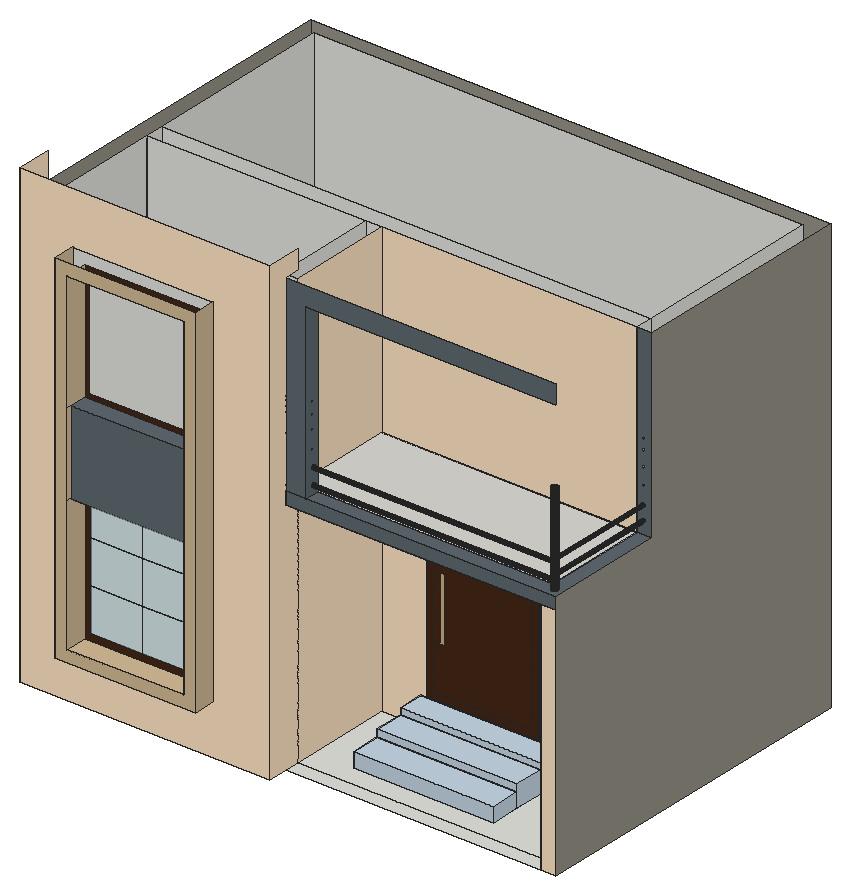
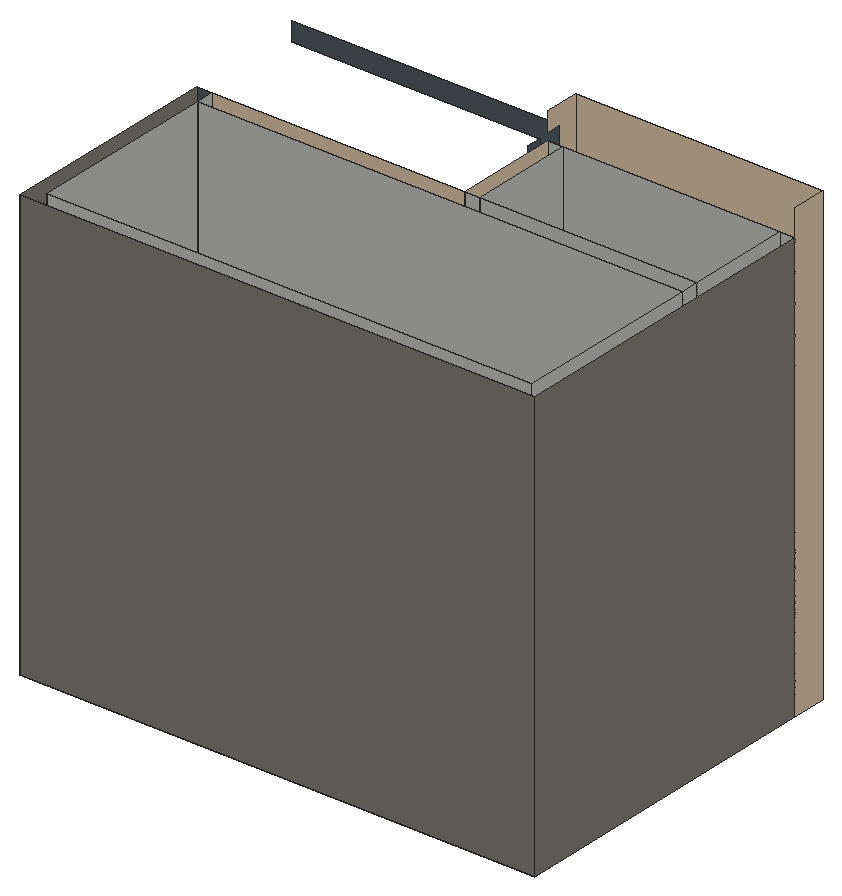
# SketchUp Ruby script. Lengths in inches.
U = 1.inch
M = Sketchup.active_model
def pt(a) = Geom::Point3d.new(a.map { |v| v * U })
def face(e, loops, mat)
  f = e.add_face(loops[0].map { |a| pt(a) })
  loops[1..].each { |l| e.add_face(l.map { |a| pt(a) }).erase! }
  f.material = f.back_material = mat if mat
  f
end
# faces: each face lists its corners as indices into pts; further lists are holes
def faces(e, pts, list, mat = nil) = list.each { |f| face(e, (f[0].is_a?(Array) ? f : [f]).map { |l| l.map { |i| pts[i] } }, mat) }
# xy, xz, yz: faces in a plane at the given z, y or x. An outline is a flat list of corners, or four numbers for a rectangle; further outlines are holes
def ring(l) = l.size == 4 ? [[l[0], l[1]], [l[2], l[1]], [l[2], l[3]], [l[0], l[3]]] : l.each_slice(2).to_a
def flat(e, list, mat, &to3) = list.each { |f| face(e, (f[0].is_a?(Array) ? f : [f]).map { |l| ring(l).map { |u, v| to3.(u, v) } }, mat) }
def xy(e, z, list, mat = nil) = flat(e, list, mat) { |x, y| [x, y, z] }
def xz(e, y, list, mat = nil) = flat(e, list, mat) { |x, z| [x, y, z] }
def yz(e, x, list, mat = nil) = flat(e, list, mat) { |y, z| [x, y, z] }
def lines(e, pts, list) = list.each { |a, b| e.add_line(pt(pts[a]), pt(pts[b])) }
# prism: a flat outline (further loops are holes) pulled along v
def prism(e, loops, v, mat = nil)
  f = face(e, loops, mat); d = Geom::Vector3d.new(v.map { |x| x * U })
  f.pushpull(f.normal.samedirection?(d) ? d.length : -d.length)
end
def box(e, o, s, mat = nil) = prism(e, [[o, [o[0] + s[0], o[1], o[2]], [o[0] + s[0], o[1] + s[1], o[2]], [o[0], o[1] + s[1], o[2]]]], [0, 0, s[2]], mat)
def at(x, y, z, deg = 0) = Geom::Transformation.translation(pt([x, y, z])) * Geom::Transformation.rotation(ORIGIN, Z_AXIS, deg.degrees)
def axes(o, x, y, z) = Geom::Transformation.new([*x, 0, *y, 0, *z, 0, *pt(o).to_a, 1])
def part(name) = M.definitions.add(name)
# library, detail: a bought-in or finely detailed component or shape, given as its bounding box
def library(name, o, s) = part(name).tap { |d| box(d.entities, o, s) }
def detail(e, o, s) = box(e.add_group.entities, o, s)
def put(e, d, t, mat = nil) = e.add_instance(d, t).tap { |i| i.material = mat if mat }
def group(e, t, mat = nil) = e.add_group.tap { |g| g.transformation = t; g.material = mat if mat }.entities
root = M.entities
M.materials.add("[0007_MistyRose]").color = [255, 228, 225]
M.materials.add("[0012_Bisque]").color = [255, 228, 196]
M.materials.add("[Color M07]").color = [58, 58, 58]
M.materials.add("[Formica Beige]").color = [211, 187, 149]
M.materials.add("[Formica Graystone]").color = [149, 146, 135]
M.materials.add("[Formica Speckled Grey]").color = [94, 105, 111]
M.materials.add("[Terrazzo Light Blue]").color = [196, 214, 227]
M.materials.add("[Terrazzo Tile Light]").color = [219, 217, 210]
M.materials.add("[Translucent Glass Safety]").color = [204, 235, 244]
M.materials["[Translucent Glass Safety]"].alpha = 0.5
M.materials.add("[Wood Floor Light]").color = [204, 176, 127]
M.materials.add("[Wood Veneer 01]").color = [68, 40, 21]
xy(root,0,[[0,11.1875,124.35,28.73],[251.5,21.1875,251.5,184.85,7.54,184.85,7.54,28.73,0,28.73,0,192.39,259.04,192.39,259.04,21.1875],[124.35,21.1875,251.5,28.73],[7.54,28.73,116.61,80.93],[116.61,28.73,124.35,80.93],
  [124.35,28.73,251.5,28.73,251.5,80.93,213.8,80.93,213.8,39.05,143.86,39.05,143.86,80.93,124.35,80.93],[143.86,39.05,213.8,53.73],[143.86,53.73,213.8,68.41],[143.86,68.41,213.8,80.93],[7.54,80.93,251.5,89.9],
  [7.54,89.9,251.5,184.85]])
xy(root,7.1875,[[143.86,39.05,213.8,53.73]],"[Terrazzo Light Blue]")
xy(root,10.75,[[143.86,53.73,213.8,68.41]],"[Terrazzo Light Blue]")
xy(root,14,[[143.86,68.41,213.8,80.93]],"[Terrazzo Light Blue]")
xy(root,14.36,[[147.19,80.93,202.75,89.9]])
xy(root,24.97,[[26.5,0,96.3125,11.1875]],"[Formica Beige]")
xy(root,30.76,[[32.29,0,90.53,11.1875]],"[Formica Beige]")
xy(root,32.27,[[213.24,80.93,244.05,89.9]])
xy(root,97.1875,[[32.29,2.3125,90.53,11.1875]],"[Formica Speckled Grey]")
xy(root,100.77,[[213.24,80.93,244.05,89.9]])
xy(root,104.26,[[147.19,80.93,202.75,89.9]])
xy(root,118.58,[[124.35,21.1875,251.5,28.73]],"[0007_MistyRose]")
xy(root,120,[[7.54,28.73,116.61,80.93],[116.61,28.73,124.35,80.93],[7.54,80.93,251.5,89.9],[7.54,89.9,251.5,184.85]])
xy(root,120,[[124.35,28.73,251.5,80.93]],"[0007_MistyRose]")
xy(root,124.5625,[[124.35,21.1875,134.6,28.73],[254.97,24.03,254.57,24.08,254.19,24.24,253.87,24.49,253.62,24.8125,253.46,25.19,253.41,25.59,253.46,26,253.62,26.375,253.87,26.7,254.19,26.95,254.57,27.1,254.97,27.16,255.38,27.1,255.75,26.95,256.08,26.7,256.33,26.375,256.48,26,256.54,25.59,256.48,25.19,256.33,24.8125,256.08,24.49,255.75,24.24,255.38,24.08],[7.54,28.73,116.61,80.93],[116.61,28.73,124.35,80.93]])
xy(root,124.5625,[[[134.6,21.1875,259.04,21.1875,259.04,80.93,251.5,80.93,251.5,28.73,134.6,28.73],[254.97,24.03,254.57,24.08,254.19,24.24,253.87,24.49,253.62,24.8125,253.46,25.19,253.41,25.59,253.46,26,253.62,26.375,253.87,26.7,254.19,26.95,254.57,27.1,254.97,27.16,255.38,27.1,255.75,26.95,256.08,26.7,256.33,26.375,256.48,26,256.54,25.59,256.48,25.19,256.33,24.8125,256.08,24.49,255.75,24.24,255.38,24.08]]],"[Formica Speckled Grey]")
xy(root,124.5625,[[124.35,28.73,251.5,80.93]],"[Terrazzo Tile Light]")
xy(root,138.74,[[32.29,2.3125,90.53,11.1875]],"[Formica Speckled Grey]")
xz(root,0,[[[26.5,24.97,96.3125,203.54],[32.29,30.76,90.53,197.75]]],"[Formica Beige]")
xz(root,2.3125,[[32.29,97.1875,90.53,138.74]],"[Formica Speckled Grey]")
xz(root,11.1875,[[[0,0,124.35,229.5],[26.5,24.97,96.3125,203.54]]],"[0012_Bisque]")
xz(root,11.1875,[[35.27,33.74,61.41,55.23],[61.41,33.74,87.54,55.23],[35.27,55.23,61.41,76.71],[61.41,55.23,87.54,76.71],[35.27,76.71,61.41,94.2],
  [61.41,76.71,87.54,94.2]],"[Translucent Glass Safety]")
xz(root,11.1875,[[[32.29,30.76,90.53,97.1875],[35.27,33.74,87.54,94.2]],[[32.29,138.74,90.53,197.75],[34.45,140.9,88.37,195.59]]],"[Wood Veneer 01]")
xz(root,21.1875,[[251.5,0,259.04,118.58]],"[0012_Bisque]")
xz(root,21.1875,[[124.35,118.58,259.04,124.5625],[124.35,124.5625,134.6,124.5625,134.6,210.1875,259.04,210.1875,259.04,219.875,124.35,219.875]],"[Formica Speckled Grey]")
xz(root,25.59,[[254.99,130.22,255.2,130.25,255.39,130.33,255.5625,130.46,255.69,130.63,255.77,130.83,255.8,131.04,255.77,131.25,255.69,131.44,255.5625,131.61,255.39,131.74,255.2,131.82,254.99,131.85,254.78,131.82,254.58,131.74,254.41,131.61,254.28,131.44,254.2,131.25,254.18,131.04,254.2,130.83,254.28,130.63,254.41,130.46,254.58,130.33,254.78,130.25],[254.99,137.16,255.2,137.19,255.39,137.27,255.5625,137.4,255.69,137.57,255.77,137.76,255.8,137.97,255.77,138.19,255.69,138.38,255.5625,138.55,255.39,138.68,255.2,138.76,254.99,138.79,254.78,138.76,254.58,138.68,254.41,138.55,254.28,138.38,254.2,138.19,254.18,137.97,254.2,137.76,254.28,137.57,254.41,137.4,254.58,137.27,254.78,137.19]])
xz(root,28.73,[[0,0,7.54,216.125],[7.54,0,116.61,120],[116.61,0,124.35,120],[124.35,118.58,251.5,120],[7.54,120,124.35,124.5625],
  [124.35,120,251.5,124.5625],[7.54,124.5625,116.61,216.125],[116.61,124.5625,124.35,216.125],[124.35,124.5625,134.6,170.34]])
xz(root,39.05,[[143.86,0,213.8,7.1875]],"[Terrazzo Light Blue]")
xz(root,53.73,[[143.86,0,213.8,7.1875]])
xz(root,53.73,[[143.86,7.1875,213.8,10.75]],"[Terrazzo Light Blue]")
xz(root,68.41,[[143.86,0,213.8,10.75]])
xz(root,68.41,[[143.86,10.75,213.8,14]],"[Terrazzo Light Blue]")
xz(root,80.93,[[7.54,0,116.61,120],[116.61,0,124.35,120],[143.86,0,213.8,14],[7.54,120,251.5,124.5625],[7.54,124.5625,116.61,216.125],
  [116.61,124.5625,124.35,216.125]])
xz(root,80.93,[[[124.35,0,143.86,0,143.86,14,213.8,14,213.8,0,251.5,0,251.5,120,124.35,120],[147.19,14.36,202.75,104.26],[213.24,32.27,244.05,100.77]],[124.35,124.5625,251.5,216.125]],"[0012_Bisque]")
xz(root,80.93,[[[251.5,124.5625,259.04,216.125],[254.99,145.96,254.78,145.99,254.58,146.07,254.41,146.2,254.28,146.37,254.2,146.5625,254.18,146.77,254.2,146.98,254.28,147.18,254.41,147.35,254.58,147.48,254.78,147.56,254.99,147.58,255.2,147.56,255.39,147.48,255.5625,147.35,255.69,147.18,255.77,146.98,255.8,146.77,255.77,146.5625,255.69,146.37,255.5625,146.2,255.39,146.07,255.2,145.99],[254.99,154.29,254.78,154.31,254.58,154.4,254.41,154.53,254.28,154.69,254.2,154.89,254.18,155.1,254.2,155.31,254.28,155.51,254.41,155.67,254.58,155.8,254.78,155.88,254.99,155.91,255.2,155.88,255.39,155.8,255.5625,155.67,255.69,155.51,255.77,155.31,255.8,155.1,255.77,154.89,255.69,154.69,255.5625,154.53,255.39,154.4,255.2,154.31],[254.99,137.16,254.78,137.19,254.58,137.27,254.41,137.4,254.28,137.57,254.2,137.76,254.18,137.97,254.2,138.19,254.28,138.38,254.41,138.55,254.58,138.68,254.78,138.76,254.99,138.79,255.2,138.76,255.39,138.68,255.5625,138.55,255.69,138.38,255.77,138.19,255.8,137.97,255.77,137.76,255.69,137.57,255.5625,137.4,255.39,137.27,255.2,137.19],[254.99,161.79,254.78,161.81,254.58,161.9,254.41,162.03,254.28,162.19,254.2,162.39,254.18,162.6,254.2,162.81,254.28,163.01,254.41,163.17,254.58,163.3,254.78,163.38,254.99,163.41,255.2,163.38,255.39,163.3,255.5625,163.17,255.69,163.01,255.77,162.81,255.8,162.6,255.77,162.39,255.69,162.19,255.5625,162.03,255.39,161.9,255.2,161.81],[254.99,130.22,254.78,130.25,254.58,130.33,254.41,130.46,254.28,130.63,254.2,130.83,254.18,131.04,254.2,131.25,254.28,131.44,254.41,131.61,254.58,131.74,254.78,131.82,254.99,131.85,255.2,131.82,255.39,131.74,255.5625,131.61,255.69,131.44,255.77,131.25,255.8,131.04,255.77,130.83,255.69,130.63,255.5625,130.46,255.39,130.33,255.2,130.25],[254.99,166.97,254.78,167,254.58,167.08,254.41,167.21,254.28,167.38,254.2,167.58,254.18,167.79,254.2,168,254.28,168.19,254.41,168.36,254.58,168.49,254.78,168.57,254.99,168.6,255.2,168.57,255.39,168.49,255.5625,168.36,255.69,168.19,255.77,168,255.8,167.79,255.77,167.58,255.69,167.38,255.5625,167.21,255.39,167.08,255.2,167]]],"[Formica Speckled Grey]")
xz(root,80.93,[[216.07,35.1,241.21,97.93]],"[Translucent Glass Safety]")
xz(root,80.93,[[153.64,40.1,156.01,72.66]],"[Wood Floor Light]")
xz(root,80.93,[[[147.19,14.36,202.75,104.26],[150.68,17.85,199.26,100.77]],[[150.68,17.85,199.26,100.77],[153.64,40.1,156.01,72.66]],[[213.24,32.27,244.05,100.77],[216.07,35.1,241.21,97.93]]],"[Wood Veneer 01]")
xz(root,89.9,[[[7.54,0,251.5,120],[147.19,14.36,202.75,104.26],[213.24,32.27,244.05,100.77]],[7.54,120,251.5,216.125]])
xz(root,184.85,[[7.54,0,251.5,120],[7.54,120,251.5,216.125]])
xz(root,192.39,[[0,0,259.04,216.125]],"[Formica Graystone]")
yz(root,0,[[11.1875,0,28.73,229.5]],"[0012_Bisque]")
yz(root,0,[[28.73,0,192.39,216.125]],"[Formica Graystone]")
yz(root,7.54,[[28.73,0,80.93,120],[80.93,0,89.9,120],[89.9,0,184.85,120],[80.93,120,89.9,216.125],[89.9,120,184.85,216.125],
  [28.73,124.5625,80.93,216.125]])
yz(root,26.5,[[0,24.97,11.1875,203.54]],"[Formica Beige]")
yz(root,32.29,[[0,30.76,11.1875,97.1875],[0,97.1875,2.3125,138.74],[0,138.74,11.1875,197.75]],"[Formica Beige]")
yz(root,90.53,[[0,30.76,11.1875,97.1875],[0,97.1875,2.3125,138.74],[0,138.74,11.1875,197.75]],"[Formica Beige]")
yz(root,96.3125,[[0,24.97,11.1875,203.54]],"[Formica Beige]")
yz(root,116.61,[[28.73,0,80.93,120],[28.73,124.5625,80.93,216.125]])
yz(root,124.35,[[21.1875,118.58,28.73,124.5625]])
yz(root,124.35,[[11.1875,0,28.73,0,28.73,118.58,21.1875,118.58,21.1875,219.875,28.73,219.875,28.73,229.5,11.1875,229.5],[28.73,0,80.93,120],[28.73,124.5625,80.93,216.125]],"[0012_Bisque]")
yz(root,124.35,[[21.1875,124.5625,28.73,170.34]],"[Color M07]")
yz(root,134.6,[[[21.1875,124.5625,28.73,210.1875],[24.83,128.51,24.62,128.54,24.42,128.62,24.25,128.75,24.125,128.91,24.04,129.11,24.01,129.32,24.04,129.53,24.125,129.73,24.25,129.9,24.42,130.02,24.62,130.11,24.83,130.13,25.04,130.11,25.23,130.02,25.4,129.9,25.53,129.73,25.61,129.53,25.64,129.32,25.61,129.11,25.53,128.91,25.4,128.75,25.23,128.62,25.04,128.54],[24.83,159.95,24.62,159.97,24.42,160.05,24.25,160.18,24.125,160.35,24.04,160.55,24.01,160.76,24.04,160.97,24.125,161.16,24.25,161.33,24.42,161.46,24.62,161.54,24.83,161.57,25.04,161.54,25.23,161.46,25.4,161.33,25.53,161.16,25.61,160.97,25.64,160.76,25.61,160.55,25.53,160.35,25.4,160.18,25.23,160.05,25.04,159.97],[24.83,136.57,24.62,136.6,24.42,136.68,24.25,136.81,24.125,136.98,24.04,137.17,24.01,137.38,24.04,137.59,24.125,137.79,24.25,137.96,24.42,138.09,24.62,138.17,24.83,138.2,25.04,138.17,25.23,138.09,25.4,137.96,25.53,137.79,25.61,137.59,25.64,137.38,25.61,137.17,25.53,136.98,25.4,136.81,25.23,136.68,25.04,136.6],[24.83,153.38,24.62,153.41,24.42,153.49,24.25,153.62,24.125,153.79,24.04,153.99,24.01,154.2,24.04,154.41,24.125,154.6,24.25,154.77,24.42,154.9,24.62,154.98,24.83,155.01,25.04,154.98,25.23,154.9,25.4,154.77,25.53,154.6,25.61,154.41,25.64,154.2,25.61,153.99,25.53,153.79,25.4,153.62,25.23,153.49,25.04,153.41],[24.83,144.63,24.62,144.66,24.42,144.74,24.25,144.87,24.125,145.04,24.04,145.24,24.01,145.45,24.04,145.66,24.125,145.85,24.25,146.02,24.42,146.15,24.62,146.23,24.83,146.26,25.04,146.23,25.23,146.15,25.4,146.02,25.53,145.85,25.61,145.66,25.64,145.45,25.61,145.24,25.53,145.04,25.4,144.87,25.23,144.74,25.04,144.66],[24.83,166.07,24.62,166.1,24.42,166.18,24.25,166.31,24.125,166.48,24.04,166.67,24.01,166.88,24.04,167.09,24.125,167.29,24.25,167.46,24.42,167.59,24.62,167.67,24.83,167.7,25.04,167.67,25.23,167.59,25.4,167.46,25.53,167.29,25.61,167.09,25.64,166.88,25.61,166.67,25.53,166.48,25.4,166.31,25.23,166.18,25.04,166.1]]],"[Formica Speckled Grey]")
yz(root,143.86,[[39.05,0,53.73,7.1875],[53.73,0,68.41,10.75],[68.41,0,80.93,14]],"[Terrazzo Light Blue]")
yz(root,147.19,[[80.93,14.36,89.9,104.26]])
yz(root,202.75,[[80.93,14.36,89.9,104.26]])
yz(root,213.24,[[80.93,32.27,89.9,100.77]])
yz(root,213.8,[[39.05,0,53.73,7.1875],[53.73,0,68.41,10.75],[68.41,0,80.93,14]],"[Terrazzo Light Blue]")
yz(root,244.05,[[80.93,32.27,89.9,100.77]])
yz(root,251.5,[[80.93,0,89.9,120],[89.9,0,184.85,120],[28.73,120,80.93,124.5625],[80.93,120,89.9,216.125],[89.9,120,184.85,216.125]])
yz(root,251.5,[[21.1875,0,28.73,118.58],[28.73,0,80.93,120]],"[0012_Bisque]")
yz(root,254.97,[[24.83,128.51,25.04,128.54,25.23,128.62,25.4,128.75,25.53,128.91,25.61,129.11,25.64,129.32,25.61,129.53,25.53,129.73,25.4,129.9,25.23,130.02,25.04,130.11,24.83,130.13,24.62,130.11,24.42,130.02,24.25,129.9,24.125,129.73,24.04,129.53,24.03,129.45,24.03,129.19,24.04,129.11,24.125,128.91,24.25,128.75,24.42,128.62,24.62,128.54],[24.03,129.19,24.03,129.45,24.01,129.32]])
yz(root,255.38,[[24.83,136.57,25.04,136.6,25.23,136.68,25.4,136.81,25.53,136.98,25.61,137.17,25.64,137.38,25.61,137.59,25.53,137.79,25.4,137.96,25.23,138.09,25.04,138.17,24.83,138.2,24.62,138.17,24.42,138.09,24.25,137.96,24.125,137.79,24.08,137.7,24.08,137.07,24.125,136.98,24.25,136.81,24.42,136.68,24.62,136.6]])
yz(root,255.38,[[24.08,137.07,24.08,137.7,24.04,137.59,24.01,137.38,24.04,137.17]],"[Color M07]")
yz(root,259.04,[[21.1875,0,192.39,0,192.39,216.125,80.93,216.125,80.93,124.5625,21.1875,124.5625]],"[Formica Graystone]")
p = [[254.57,24.08,124.5625],[254.97,24.03,124.5625],[254.97,24.03,129.19],[254.97,24.03,129.45],[254.97,24.03,170.34],[254.57,24.08,170.34],
  [254.57,24.08,145.76],[254.57,24.08,145.13],[255.38,24.08,124.5625],[255.38,24.08,137.07],[255.38,24.08,137.7],[255.38,24.08,170.34],
  [254.19,24.24,124.5625],[254.19,24.24,170.34],[254.19,24.24,154.75],[254.19,24.24,153.64],[255.75,24.24,124.5625],[255.75,24.24,170.34],
  [253.87,24.49,124.5625],[253.87,24.49,170.34],[253.87,24.49,167.62],[253.87,24.49,166.15],[256.08,24.49,124.5625],[256.08,24.49,170.34],
  [253.62,24.8125,124.5625],[253.62,24.8125,170.34],[256.33,24.8125,124.5625],[256.33,24.8125,170.34],[253.46,25.19,124.5625],[253.46,25.19,170.34],
  [256.48,25.19,124.5625],[256.48,25.19,170.34],[253.41,25.59,124.5625],[253.41,25.59,170.34],[256.54,25.59,124.5625],[256.54,25.59,170.34],
  [253.46,26,124.5625],[253.46,26,170.34],[256.48,26,124.5625],[256.48,26,170.34],[253.62,26.375,124.5625],[253.62,26.375,170.34],
  [256.33,26.375,124.5625],[256.33,26.375,170.34],[253.87,26.7,124.5625],[253.87,26.7,170.34],[256.08,26.7,124.5625],[256.08,26.7,170.34],
  [254.19,26.95,124.5625],[254.19,26.95,170.34],[255.75,26.95,124.5625],[255.75,26.95,170.34],[254.57,27.1,124.5625],[254.57,27.1,170.34],
  [255.38,27.1,124.5625],[255.38,27.1,170.34],[254.97,27.16,124.5625],[254.97,27.16,170.34],[254.97,24.42,128.62],[134.6,24.42,128.62],
  [134.6,24.62,128.54],[254.97,24.62,128.54],[134.6,24.83,128.51],[254.97,24.83,128.51],[134.6,25.04,128.54],[254.97,25.04,128.54],
  [134.6,25.23,128.62],[254.97,25.23,128.62],[254.97,24.25,128.75],[134.6,24.25,128.75],[134.6,25.4,128.75],[254.97,25.4,128.75],
  [254.97,24.125,128.91],[134.6,24.125,128.91],[134.6,25.53,128.91],[254.97,25.53,128.91],[254.97,24.04,129.11],[134.6,24.04,129.11],
  [134.6,25.61,129.11],[254.97,25.61,129.11],[254.97,24.01,129.32],[134.6,24.01,129.32],[134.6,25.64,129.32],[254.97,25.64,129.32],
  [254.97,24.04,129.53],[134.6,24.04,129.53],[134.6,25.61,129.53],[254.97,25.61,129.53],[254.97,24.125,129.73],[134.6,24.125,129.73],
  [134.6,25.53,129.73],[254.97,25.53,129.73],[254.97,24.25,129.9],[134.6,24.25,129.9],[134.6,25.4,129.9],[254.97,25.4,129.9],
  [254.97,24.42,130.02],[134.6,24.42,130.02],[134.6,25.23,130.02],[254.97,25.23,130.02],[254.97,24.62,130.11],[134.6,24.62,130.11],
  [134.6,25.04,130.11],[254.97,25.04,130.11],[254.97,24.83,130.13],[134.6,24.83,130.13],[254.78,80.93,130.25],[254.99,80.93,130.22],
  [254.99,25.59,130.22],[254.78,25.59,130.25],[255.2,80.93,130.25],[255.2,25.59,130.25],[254.41,80.93,130.46],[254.58,80.93,130.33],
  [254.58,25.59,130.33],[254.41,25.59,130.46],[255.39,80.93,130.33],[255.39,25.59,130.33],[255.5625,80.93,130.46],[255.5625,25.59,130.46],
  [254.28,80.93,130.63],[254.28,25.59,130.63],[255.69,80.93,130.63],[255.69,25.59,130.63],[254.2,80.93,130.83],[254.2,25.59,130.83],
  [255.77,80.93,130.83],[255.77,25.59,130.83],[254.18,80.93,131.04],[254.18,25.59,131.04],[255.8,80.93,131.04],[255.8,25.59,131.04],
  [254.2,80.93,131.25],[254.2,25.59,131.25],[255.77,80.93,131.25],[255.77,25.59,131.25],[254.28,80.93,131.44],[254.28,25.59,131.44],
  [255.69,80.93,131.44],[255.69,25.59,131.44],[254.41,80.93,131.61],[254.41,25.59,131.61],[255.5625,80.93,131.61],[255.5625,25.59,131.61],
  [254.58,80.93,131.74],[254.58,25.59,131.74],[255.39,80.93,131.74],[255.39,25.59,131.74],[254.78,80.93,131.82],[254.78,25.59,131.82],
  [255.2,80.93,131.82],[255.2,25.59,131.82],[254.99,80.93,131.85],[254.99,25.59,131.85],[255.38,24.42,136.68],[134.6,24.42,136.68],
  [134.6,24.62,136.6],[255.38,24.62,136.6],[134.6,24.83,136.57],[255.38,24.83,136.57],[134.6,25.04,136.6],[255.38,25.04,136.6],
  [134.6,25.23,136.68],[255.38,25.23,136.68],[255.38,24.25,136.81],[134.6,24.25,136.81],[134.6,25.4,136.81],[255.38,25.4,136.81],
  [255.38,24.125,136.98],[134.6,24.125,136.98],[134.6,25.53,136.98],[255.38,25.53,136.98],[255.38,24.04,137.17],[134.6,24.04,137.17],
  [134.6,25.61,137.17],[255.38,25.61,137.17],[255.38,24.01,137.38],[134.6,24.01,137.38],[134.6,25.64,137.38],[255.38,25.64,137.38],
  [254.58,80.93,137.27],[254.78,80.93,137.19],[254.78,25.59,137.19],[254.58,25.59,137.27],[254.99,80.93,137.16],[254.99,25.59,137.16],
  [255.2,80.93,137.19],[255.2,25.59,137.19],[255.39,80.93,137.27],[255.39,25.59,137.27],[254.41,80.93,137.4],[254.41,25.59,137.4],
  [255.5625,80.93,137.4],[255.5625,25.59,137.4],[255.38,24.04,137.59],[134.6,24.04,137.59],[134.6,25.61,137.59],[255.38,25.61,137.59],
  [254.28,80.93,137.57],[254.28,25.59,137.57],[255.69,80.93,137.57],[255.69,25.59,137.57],[255.38,24.125,137.79],[134.6,24.125,137.79],
  [134.6,25.53,137.79],[255.38,25.53,137.79],[254.2,80.93,137.76],[254.2,25.59,137.76],[255.77,80.93,137.76],[255.77,25.59,137.76],
  [255.38,24.25,137.96],[134.6,24.25,137.96],[134.6,25.4,137.96],[255.38,25.4,137.96],[254.18,80.93,137.97],[254.18,25.59,137.97],
  [255.8,80.93,137.97],[255.8,25.59,137.97],[255.38,24.42,138.09],[134.6,24.42,138.09],[134.6,25.23,138.09],[255.38,25.23,138.09],
  [254.2,80.93,138.19],[254.2,25.59,138.19],[255.77,80.93,138.19],[255.77,25.59,138.19],[255.38,24.62,138.17],[134.6,24.62,138.17],
  [134.6,25.04,138.17],[255.38,25.04,138.17],[255.38,24.83,138.2],[134.6,24.83,138.2],[254.28,80.93,138.38],[254.28,25.59,138.38],
  [255.69,80.93,138.38],[255.69,25.59,138.38],[254.41,80.93,138.55],[254.41,25.59,138.55],[255.5625,80.93,138.55],[255.5625,25.59,138.55],
  [254.58,80.93,138.68],[254.58,25.59,138.68],[255.39,80.93,138.68],[255.39,25.59,138.68],[254.78,80.93,138.76],[254.78,25.59,138.76],
  [255.2,80.93,138.76],[255.2,25.59,138.76],[254.99,80.93,138.79],[254.99,25.59,138.79],[116.61,28.73,120],[116.61,80.93,124.5625]]
faces(root,p,[[0,1,2,3,4,5,6,7],[1,8,9,10,11,4,3,2],[12,0,7,6,5,13,14,15],[8,16,17,11,10,9],[18,12,15,14,13,19,20,21],[16,22,23,17],[24,18,21,20,19,25],[22,26,27,23],
  [28,24,25,29],[26,30,31,27],[32,28,29,33],[30,34,35,31],[36,32,33,37],[34,38,39,35],[40,36,37,41],[38,42,43,39],
  [44,40,41,45],[42,46,47,43],[48,44,45,49],[46,50,51,47],[52,48,49,53],[50,54,55,51],[56,52,53,57],[54,56,57,55],
  [58,59,60,61],[61,60,62,63],[63,62,64,65],[65,64,66,67],[68,69,59,58],[67,66,70,71],[72,73,69,68],[71,70,74,75],
  [76,77,73,72],[75,74,78,79],[80,81,77,76,2],[79,78,82,83],[84,85,81,80,3],[83,82,86,87],[88,89,85,84],[87,86,90,91],
  [92,93,89,88],[91,90,94,95],[96,97,93,92],[95,94,98,99],[100,101,97,96],[99,98,102,103],[104,105,101,100],[103,102,105,104],
  [106,107,108,109],[107,110,111,108],[112,113,114,115],[113,106,109,114],[110,116,117,111],[116,118,119,117],[120,112,115,121],[118,122,123,119],
  [124,120,121,125],[122,126,127,123],[128,124,125,129],[126,130,131,127],[132,128,129,133],[130,134,135,131],[136,132,133,137],[134,138,139,135],
  [140,136,137,141],[138,142,143,139],[144,140,141,145],[142,146,147,143],[148,144,145,149],[146,150,151,147],[152,148,149,153],[150,152,153,151],
  [154,155,156,157],[157,156,158,159],[159,158,160,161],[161,160,162,163],[164,165,155,154],[163,162,166,167],[168,169,165,164],[167,166,170,171],
  [172,173,169,168,9],[171,170,174,175],[176,177,173,172],[175,174,178,179],[180,181,182,183],[181,184,185,182],[184,186,187,185],[186,188,189,187],
  [190,180,183,191],[188,192,193,189],[194,195,177,176],[179,178,196,197],[198,190,191,199],[192,200,201,193],[202,203,195,194,10],[197,196,204,205],
  [206,198,199,207],[200,208,209,201],[210,211,203,202],[205,204,212,213],[214,206,207,215],[208,216,217,209],[218,219,211,210],[213,212,220,221],
  [222,214,215,223],[216,224,225,217],[226,227,219,218],[221,220,228,229],[230,231,227,226],[229,228,231,230],[232,222,223,233],[224,234,235,225],
  [236,232,233,237],[234,238,239,235],[240,236,237,241],[238,242,243,239],[244,240,241,245],[242,246,247,243],[248,244,245,249],[246,248,249,247]],"[Color M07]")
lines(root,p,[[250,251]])
